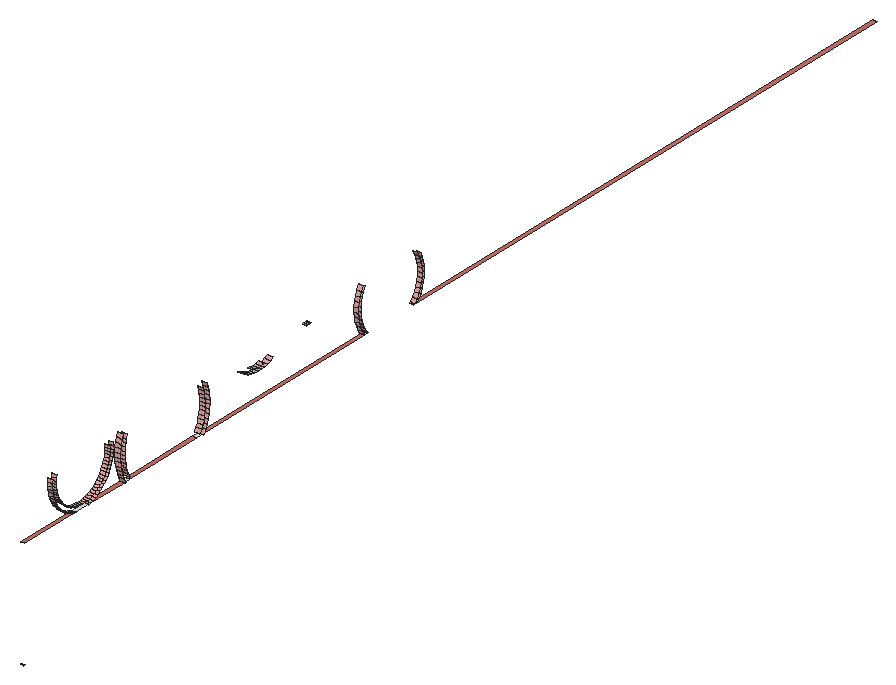
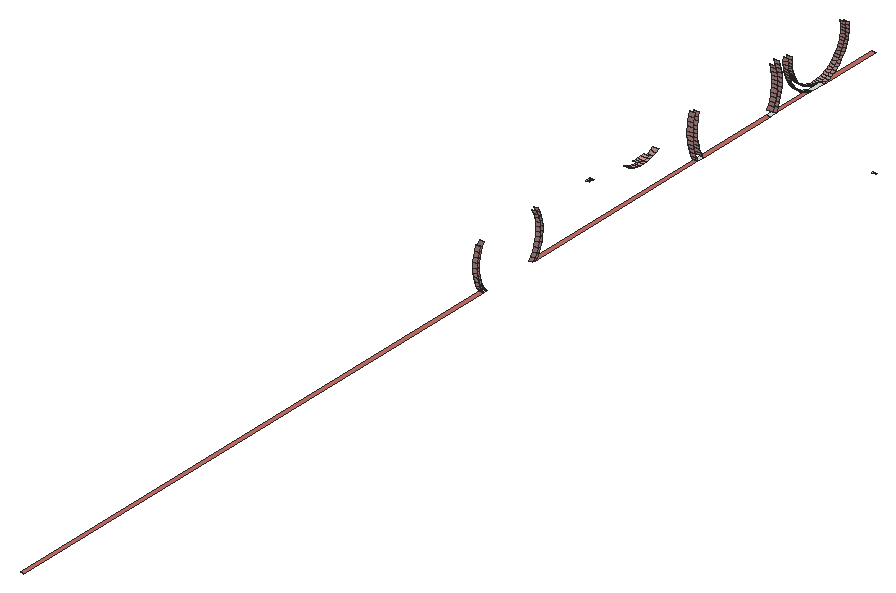
# SketchUp Ruby script. Lengths in inches.
U = 1.inch
M = Sketchup.active_model
def pt(a) = Geom::Point3d.new(a.map { |v| v * U })
def face(e, loops, mat)
  f = e.add_face(loops[0].map { |a| pt(a) })
  loops[1..].each { |l| e.add_face(l.map { |a| pt(a) }).erase! }
  f.material = f.back_material = mat if mat
  f
end
# faces: each face lists its corners as indices into pts; further lists are holes
def faces(e, pts, list, mat = nil) = list.each { |f| face(e, (f[0].is_a?(Array) ? f : [f]).map { |l| l.map { |i| pts[i] } }, mat) }
# xy, xz, yz: faces in a plane at the given z, y or x. An outline is a flat list of corners, or four numbers for a rectangle; further outlines are holes
def ring(l) = l.size == 4 ? [[l[0], l[1]], [l[2], l[1]], [l[2], l[3]], [l[0], l[3]]] : l.each_slice(2).to_a
def flat(e, list, mat, &to3) = list.each { |f| face(e, (f[0].is_a?(Array) ? f : [f]).map { |l| ring(l).map { |u, v| to3.(u, v) } }, mat) }
def xy(e, z, list, mat = nil) = flat(e, list, mat) { |x, y| [x, y, z] }
def xz(e, y, list, mat = nil) = flat(e, list, mat) { |x, z| [x, y, z] }
def yz(e, x, list, mat = nil) = flat(e, list, mat) { |y, z| [x, y, z] }
def lines(e, pts, list) = list.each { |a, b| e.add_line(pt(pts[a]), pt(pts[b])) }
# prism: a flat outline (further loops are holes) pulled along v
def prism(e, loops, v, mat = nil)
  f = face(e, loops, mat); d = Geom::Vector3d.new(v.map { |x| x * U })
  f.pushpull(f.normal.samedirection?(d) ? d.length : -d.length)
end
def box(e, o, s, mat = nil) = prism(e, [[o, [o[0] + s[0], o[1], o[2]], [o[0] + s[0], o[1] + s[1], o[2]], [o[0], o[1] + s[1], o[2]]]], [0, 0, s[2]], mat)
def at(x, y, z, deg = 0) = Geom::Transformation.translation(pt([x, y, z])) * Geom::Transformation.rotation(ORIGIN, Z_AXIS, deg.degrees)
def axes(o, x, y, z) = Geom::Transformation.new([*x, 0, *y, 0, *z, 0, *pt(o).to_a, 1])
def part(name) = M.definitions.add(name)
# library, detail: a bought-in or finely detailed component or shape, given as its bounding box
def library(name, o, s) = part(name).tap { |d| box(d.entities, o, s) }
def detail(e, o, s) = box(e.add_group.entities, o, s)
def put(e, d, t, mat = nil) = e.add_instance(d, t).tap { |i| i.material = mat if mat }
def group(e, t, mat = nil) = e.add_group.tap { |g| g.transformation = t; g.material = mat if mat }.entities
root = M.entities
M.materials.add("Generic").color = [224, 169, 169]
M.materials.add("[Wood Floor Dark]").color = [198, 114, 106]
xy(root,0,[[10.6875,0,12.375,0.4375]])
xy(root,46.5,[[10.6875,27.54,12.375,34.125],[10.6875,53.23,12.375,56.0625],[10.6875,91.96,12.375,94.93],[10.6875,181.21,12.375,182.81],[10.6875,207.45,12.375,209.04]])
xy(root,46.5,[[10.6875,0.4375,12.375,27.54],[10.6875,34.125,12.375,53.23],[10.6875,56.0625,12.375,91.96],[10.6875,94.93,12.375,181.21],[10.6875,209.04,12.375,453.375]],"[Wood Floor Dark]")
xz(root,14.55,[[10.6875,61.68,12.625,63.06]],"Generic")
xz(root,45.07,[[10.6875,61.9,12.625,63.11]],"Generic")
xz(root,50.33,[[10.6875,56.96,12.9375,58.74]],"Generic")
p = [[10.6875,26.8,46.66],[10.6875,27.54,46.5],[12.375,27.54,46.5],[12.625,27.54,46.5],[12.625,26.8,46.66],[10.6875,34.125,46.5],
  [10.6875,35.01,46.69],[12.625,35.01,46.69],[12.625,34.125,46.5],[12.375,34.125,46.5],[10.6875,94.96,46.54],[10.6875,95.8,48.26],
  [12.9375,95.8,48.26],[12.9375,94.96,46.54],[10.6875,180.86,46.93],[10.6875,181.21,46.5],[12.375,181.21,46.5],[12.375,180.86,46.93],
  [10.6875,182.81,46.5],[10.6875,181.875,47.65],[12.375,181.875,47.65],[12.375,182.81,46.5],[10.6875,207.7,46.77],[10.6875,207.45,46.5],
  [12.375,207.45,46.5],[12.375,207.7,46.77],[10.6875,209.04,46.5],[10.6875,209.84,47.59],[12.375,209.84,47.59],[12.375,209.04,46.5],
  [10.6875,25.47,47.06],[12.625,25.47,47.06],[10.6875,36.33,47.11],[12.625,36.33,47.11],[10.6875,52.32,48.33],[10.6875,53.12,46.68],
  [12.9375,53.12,46.68],[12.9375,52.32,48.33],[10.6875,208.8,48.27],[12.375,208.8,48.27],[10.6875,179.79,48.62],[12.375,179.79,48.62],
  [10.6875,24.1875,47.57],[12.625,24.1875,47.57],[10.6875,37.61,47.625],[12.625,37.61,47.625],[10.6875,22.95,48.18],[12.625,22.95,48.18],
  [10.6875,38.84,48.25],[12.625,38.84,48.25],[10.6875,210.84,49.33],[12.375,210.84,49.33],[10.6875,180.875,49.23],[12.375,180.875,49.23],
  [10.6875,55.2,47.85],[10.6875,54.5,49.29],[12.9375,54.5,49.29],[12.9375,55.2,47.85],[10.6875,93.62,49.23],[10.6875,92.92,47.79],
  [12.9375,92.92,47.79],[12.9375,93.62,49.23],[10.6875,21.77,48.9],[12.625,21.77,48.9],[10.6875,29.6875,48.24],[10.6875,28.49,48.39],
  [12.625,28.49,48.39],[12.625,29.6875,48.24],[10.6875,30.9,48.2],[12.625,30.9,48.2],[10.6875,32.1,48.25],[12.625,32.1,48.25],
  [10.6875,33.3,48.41],[12.625,33.3,48.41],[10.6875,40.02,48.99],[12.625,40.02,48.99],[10.6875,51.66,49.99],[12.9375,51.66,49.99],
  [10.6875,96.46,49.91],[12.9375,96.46,49.91],[10.6875,209.72,49.89],[12.375,209.72,49.89],[10.6875,27.3,48.64],[12.625,27.3,48.64],
  [10.6875,34.48,48.67],[12.625,34.48,48.67],[10.6875,26.14,48.99],[12.625,26.14,48.99],[10.6875,178.91,50.42],[12.375,178.91,50.42],
  [10.6875,35.64,49.03],[12.625,35.64,49.03],[10.6875,20.65,49.72],[12.625,20.65,49.72],[10.6875,25.02,49.43],[12.625,25.02,49.43],
  [10.6875,36.76,49.49],[12.625,36.76,49.49],[10.6875,41.125,49.8125],[12.625,41.125,49.8125],[10.6875,94.21,50.71],[12.9375,94.21,50.71],
  [10.6875,180.06,50.9],[12.375,180.06,50.9],[10.6875,53.91,50.78],[12.9375,53.91,50.78],[10.6875,211.63,51.17],[12.375,211.63,51.17],
  [10.6875,23.9375,49.97],[12.625,23.9375,49.97],[10.6875,37.84,50.04],[12.625,37.84,50.04],[10.6875,19.61,50.63],[12.625,19.61,50.63],
  [10.6875,42.16,50.73],[12.625,42.16,50.73],[10.6875,96.99,51.61],[12.9375,96.99,51.61],[10.6875,210.46,51.6],[12.375,210.46,51.6],
  [10.6875,22.9,50.6],[12.625,22.9,50.6],[10.6875,38.86,50.67],[12.625,38.86,50.67],[10.6875,51.13,51.69],[12.9375,51.13,51.69],
  [10.6875,178.25,52.32],[12.375,178.25,52.32],[10.6875,18.65,51.625],[12.625,18.65,51.625],[10.6875,21.93,51.32],[12.625,21.93,51.32],
  [10.6875,39.83,51.4],[12.625,39.83,51.4],[10.6875,43.11,51.73],[12.625,43.11,51.73],[10.6875,94.69,52.24],[12.9375,94.69,52.24],
  [10.6875,53.4375,52.31],[12.9375,53.4375,52.31],[10.6875,179.45,52.66],[12.375,179.45,52.66],[10.6875,212.21,53.09],[12.375,212.21,53.09],
  [10.6875,21.02,52.11],[12.625,21.02,52.11],[10.6875,40.74,52.2],[12.625,40.74,52.2],[10.6875,17.77,52.7],[12.625,17.77,52.7],
  [10.6875,97.4,53.35],[12.9375,97.4,53.35],[10.6875,210.99,53.38],[12.375,210.99,53.38],[10.6875,43.98,52.8125],[12.625,43.98,52.8125],
  [10.6875,50.73,53.42],[12.9375,50.73,53.42],[10.6875,20.18,52.98],[12.625,20.18,52.98],[10.6875,41.57,53.08],[12.625,41.57,53.08],
  [10.6875,95.06,53.8],[12.9375,95.06,53.8],[10.6875,53.08,53.87],[12.9375,53.08,53.87],[10.6875,177.81,54.27],[12.375,177.81,54.27],
  [10.6875,16.99,53.84],[12.625,16.99,53.84],[10.6875,179.04,54.48],[12.375,179.04,54.48],[10.6875,44.75,53.96],[12.625,44.75,53.96],
  [10.6875,19.41,53.92],[12.625,19.41,53.92],[10.6875,42.33,54.02],[12.625,42.33,54.02],[10.6875,212.56,55.07],[12.375,212.56,55.07],
  [10.6875,97.67,55.1],[12.9375,97.67,55.1],[10.6875,50.47,55.18],[12.9375,50.47,55.18],[10.6875,211.32,55.22],[12.375,211.32,55.22],
  [10.6875,16.3125,55.04],[12.625,16.3125,55.04],[10.6875,95.3,55.38],[12.9375,95.3,55.38],[10.6875,18.73,54.92],[12.625,18.73,54.92],
  [10.6875,52.84,55.45],[12.9375,52.84,55.45],[10.6875,43,55.03],[12.625,43,55.03],[10.6875,45.42,55.17],[12.625,45.42,55.17],
  [10.6875,177.59,56.27],[12.375,177.59,56.27],[10.6875,178.84,56.33],[12.375,178.84,56.33],[10.6875,18.14,55.97],[12.625,18.14,55.97],
  [10.6875,15.74,56.3],[12.625,15.74,56.3],[10.6875,43.58,56.09],[12.625,43.58,56.09],[10.6875,97.8125,56.88],[12.9375,97.8125,56.88],
  [10.6875,212.6875,57.07],[12.375,212.6875,57.07],[10.6875,45.98,56.4375],[12.625,45.98,56.4375],[10.6875,50.33,56.96],[12.9375,50.33,56.96],
  [10.6875,211.4375,57.07],[12.375,211.4375,57.07],[10.6875,95.43,56.98],[12.9375,95.43,56.98],[10.6875,52.72,57.05],[12.9375,52.72,57.05],
  [10.6875,17.63,57.07],[12.625,17.63,57.07],[10.6875,44.08,57.19],[12.625,44.08,57.19],[10.6875,15.27,57.6],[12.625,15.27,57.6],
  [10.6875,177.6,58.27],[12.375,177.6,58.27],[10.6875,178.85,58.19],[12.375,178.85,58.19],[10.6875,46.43,57.74],[12.625,46.43,57.74],
  [10.6875,97.82,58.66],[12.9375,97.82,58.66],[10.6875,52.71,58.65],[12.9375,52.71,58.65],[10.6875,95.4375,58.58],[12.9375,95.4375,58.58],
  [10.6875,17.23,58.21],[12.625,17.23,58.21],[10.6875,211.34,58.93],[12.375,211.34,58.93],[10.6875,212.58,59.07],[12.375,212.58,59.07],
  [10.6875,44.48,58.33],[12.625,44.48,58.33],[10.6875,14.92,58.94],[12.625,14.92,58.94],[10.6875,46.78,59.08],[12.625,46.78,59.08],
  [10.6875,122.16,58.18],[10.6875,123.83,58.04],[12.9375,123.83,58.04],[12.9375,122.16,58.18],[10.6875,125.5,58.09],[12.9375,125.5,58.09],
  [10.6875,127.15,58.33],[12.9375,127.15,58.33],[10.6875,16.92,59.38],[12.625,16.92,59.38],[10.6875,120.52,58.51],[12.9375,120.52,58.51],
  [10.6875,179.07,60.04],[12.375,179.07,60.04],[10.6875,44.78,59.51],[12.625,44.78,59.51],[10.6875,128.76,58.76],[12.9375,128.76,58.76],
  [10.6875,177.84,60.26],[12.375,177.84,60.26],[10.6875,118.93,59.02],[12.9375,118.93,59.02],[10.6875,95.32,60.18],[12.9375,95.32,60.18],
  [10.6875,50.46,60.51],[10.6875,50.33,58.74],[12.9375,50.33,58.74],[12.9375,50.46,60.51],[10.6875,52.83,60.25],[12.9375,52.83,60.25],
  [10.6875,97.7,60.4375],[12.9375,97.7,60.4375],[10.6875,130.32,59.36],[12.9375,130.32,59.36],[10.6875,14.68,60.3],[12.625,14.68,60.3],
  [10.6875,211.04,60.77],[12.375,211.04,60.77],[10.6875,117.41,59.71],[12.9375,117.41,59.71],[10.6875,47,60.45],[12.625,47,60.45],
  [10.6875,212.25,61.05],[12.375,212.25,61.05],[10.6875,16.71,60.57],[12.625,16.71,60.57],[10.6875,131.8,60.15],[12.9375,131.8,60.15],
  [10.6875,44.97,60.7],[12.625,44.97,60.7],[10.6875,123.87,59.48],[10.6875,122.36,59.61],[12.9375,122.36,59.61],[12.9375,123.87,59.48],
  [10.6875,125.37,59.53],[12.9375,125.37,59.53],[10.6875,126.86,59.74],[12.9375,126.86,59.74],[10.6875,120.89,59.91],[12.9375,120.89,59.91],
  [10.6875,115.98,60.57],[12.9375,115.98,60.57],[10.6875,179.5,61.85],[12.375,179.5,61.85],[10.6875,53.07,61.83],[12.9375,53.07,61.83],
  [10.6875,95.09,61.76],[12.9375,95.09,61.76],[10.6875,14.55,61.68],[12.625,14.55,61.68],[10.6875,178.31,62.21],[12.375,178.31,62.21],
  [10.6875,47.12,61.83],[12.625,47.12,61.83],[10.6875,97.44,62.2],[12.9375,97.44,62.2],[10.6875,50.72,62.27],[12.9375,50.72,62.27],
  [10.6875,16.6,61.78],[12.625,16.6,61.78],[10.6875,45.07,61.9],[12.625,45.07,61.9],[10.6875,210.52,62.5625],[12.375,210.52,62.5625],
  [10.6875,211.7,62.97],[12.375,211.7,62.97],[10.6875,16.59,62.99],[12.625,16.59,62.99],[10.6875,47.11,63.21],[12.625,47.11,63.21],
  [10.6875,53.42,63.39],[12.9375,53.42,63.39],[10.6875,94.74,63.33],[12.9375,94.74,63.33],[10.6875,180.14,63.6],[12.375,180.14,63.6],
  [10.6875,97.05,63.93],[12.9375,97.05,63.93],[10.6875,178.99,64.1],[12.375,178.99,64.1],[10.6875,51.12,64.01],[12.9375,51.12,64.01],
  [10.6875,209.81,64.28],[12.375,209.81,64.28],[10.6875,16.6875,64.19],[12.625,16.6875,64.19],[10.6875,210.93,64.82],[12.375,210.93,64.82],
  [10.6875,14.66,64.44],[10.6875,14.55,63.06],[12.625,14.55,63.06],[12.625,14.66,64.44],[10.6875,44.96,64.32],[10.6875,45.07,63.11],
  [12.625,45.07,63.11],[12.625,44.96,64.32],[10.6875,46.99,64.59],[12.625,46.99,64.59],[10.6875,94.28,64.86],[12.9375,94.28,64.86],
  [10.6875,53.89,64.92],[12.9375,53.89,64.92],[10.6875,180.97,65.27],[12.375,180.97,65.27],[10.6875,150.95,63.83],[10.6875,150.16,63.7],
  [12.375,150.16,63.7],[12.375,150.95,63.83],[10.6875,151.76,63.87],[12.375,151.76,63.87],[10.6875,152.5625,63.81],[12.375,152.5625,63.81],
  [10.6875,96.53,65.64],[12.9375,96.53,65.64],[10.6875,51.64,65.71],[12.9375,51.64,65.71],[10.6875,179.89,65.89],[12.375,179.89,65.89],
  [10.6875,16.89,65.39],[12.625,16.89,65.39],[10.6875,208.9,65.91],[12.375,208.9,65.91]]
faces(root,p,[[0,1,2,3,4],[5,6,7,8,9],[10,11,12,13],[14,15,16,17],[18,19,20,21],[22,23,24,25],[26,27,28,29],[30,0,4,31],
  [6,32,33,7],[34,35,36,37],[38,22,25,39],[40,14,17,41],[42,30,31,43],[32,44,45,33],[46,42,43,47],[44,48,49,45],
  [27,50,51,28],[19,52,53,20],[54,55,56,57],[58,59,60,61],[62,46,47,63],[64,65,66,67],[68,64,67,69],[70,68,69,71],
  [72,70,71,73],[48,74,75,49],[76,34,37,77],[11,78,79,12],[80,38,39,81],[65,82,83,66],[84,72,73,85],[82,86,87,83],
  [88,40,41,89],[90,84,85,91],[92,62,63,93],[86,94,95,87],[96,90,91,97],[74,98,99,75],[100,58,61,101],[52,102,103,53],
  [55,104,105,56],[50,106,107,51],[94,108,109,95],[110,96,97,111],[112,92,93,113],[98,114,115,99],[78,116,117,79],[118,80,81,119],
  [108,120,121,109],[122,110,111,123],[124,76,77,125],[126,88,89,127],[128,112,113,129],[120,130,131,121],[132,122,123,133],[114,134,135,115],
  [136,100,101,137],[104,138,139,105],[102,140,141,103],[106,142,143,107],[130,144,145,131],[146,132,133,147],[148,128,129,149],[116,150,151,117],
  [152,118,119,153],[134,154,155,135],[156,124,125,157],[144,158,159,145],[160,146,147,161],[162,136,137,163],[138,164,165,139],[166,126,127,167],
  [168,148,149,169],[140,170,171,141],[154,172,173,155],[158,174,175,159],[176,160,161,177],[142,178,179,143],[150,180,181,151],[182,156,157,183],
  [184,152,153,185],[186,168,169,187],[188,162,163,189],[174,190,191,175],[164,192,193,165],[194,176,177,195],[172,196,197,173],[198,166,167,199],
  [170,200,201,171],[190,202,203,191],[204,186,187,205],[206,194,195,207],[180,208,209,181],[178,210,211,179],[196,212,213,197],[214,182,183,215],
  [216,184,185,217],[218,188,189,219],[192,220,221,193],[202,222,223,203],[224,206,207,225],[226,204,205,227],[228,198,199,229],[200,230,231,201],
  [212,232,233,213],[208,234,235,209],[220,236,237,221],[238,218,219,239],[222,240,241,223],[242,216,217,243],[210,244,245,211],[246,224,225,247],
  [248,226,227,249],[232,250,251,233],[252,253,254,255],[253,256,257,254],[256,258,259,257],[240,260,261,241],[262,252,255,263],[230,264,265,231],
  [266,246,247,267],[258,268,269,259],[270,228,229,271],[272,262,263,273],[274,238,239,275],[276,277,278,279],[236,280,281,237],[234,282,283,235],
  [268,284,285,269],[286,248,249,287],[288,242,243,289],[290,272,273,291],[250,292,293,251],[244,294,295,245],[260,296,297,261],[284,298,299,285],
  [300,266,267,301],[302,303,304,305],[306,302,305,307],[308,306,307,309],[303,310,311,304],[312,290,291,313],[264,314,315,265],[280,316,317,281],
  [318,274,275,319],[320,286,287,321],[322,270,271,323],[292,324,325,293],[282,326,327,283],[328,276,279,329],[296,330,331,297],[332,300,301,333],
  [334,288,289,335],[294,336,337,295],[330,338,339,331],[324,340,341,325],[316,342,343,317],[344,318,319,345],[314,346,347,315],[326,348,349,327],
  [350,322,323,351],[352,328,329,353],[354,334,335,355],[338,356,357,339],[336,358,359,337],[360,361,362,363],[364,365,366,367],[340,368,369,341],
  [370,344,345,371],[342,372,373,343],[346,374,375,347],[376,377,378,379],[380,376,379,381],[382,380,381,383],[348,384,385,349],[386,352,353,387],
  [388,350,351,389],[356,390,391,357],[392,354,355,393]],"Generic")
